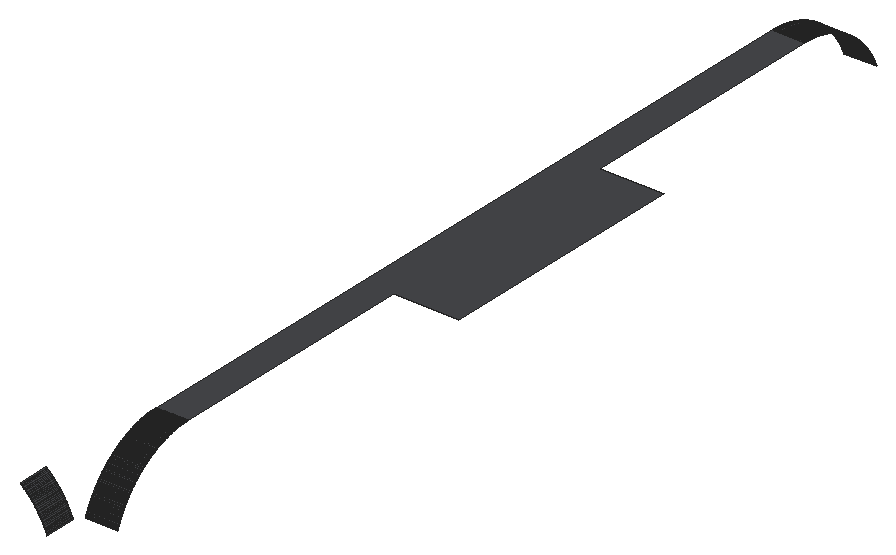
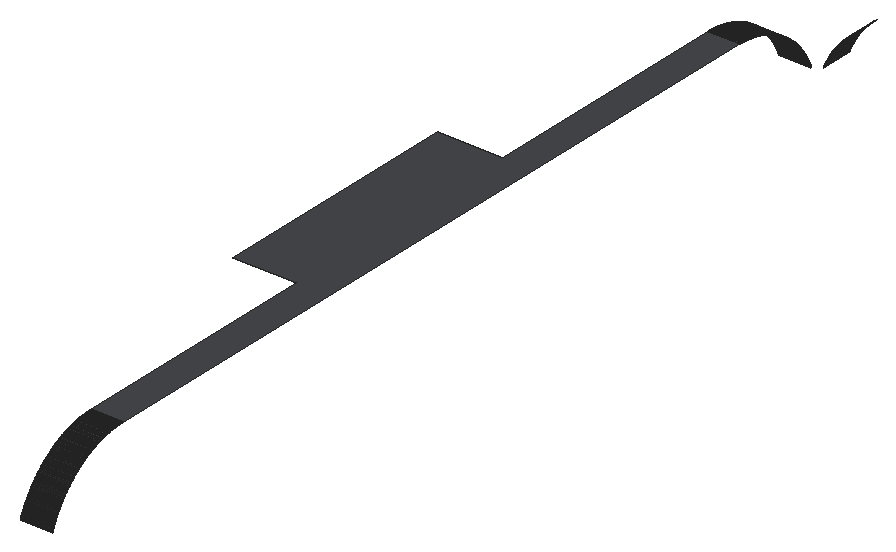
# SketchUp Ruby script. Lengths in inches.
U = 1.inch
M = Sketchup.active_model
def pt(a) = Geom::Point3d.new(a.map { |v| v * U })
def face(e, loops, mat)
  f = e.add_face(loops[0].map { |a| pt(a) })
  loops[1..].each { |l| e.add_face(l.map { |a| pt(a) }).erase! }
  f.material = f.back_material = mat if mat
  f
end
# faces: each face lists its corners as indices into pts; further lists are holes
def faces(e, pts, list, mat = nil) = list.each { |f| face(e, (f[0].is_a?(Array) ? f : [f]).map { |l| l.map { |i| pts[i] } }, mat) }
# xy, xz, yz: faces in a plane at the given z, y or x. An outline is a flat list of corners, or four numbers for a rectangle; further outlines are holes
def ring(l) = l.size == 4 ? [[l[0], l[1]], [l[2], l[1]], [l[2], l[3]], [l[0], l[3]]] : l.each_slice(2).to_a
def flat(e, list, mat, &to3) = list.each { |f| face(e, (f[0].is_a?(Array) ? f : [f]).map { |l| ring(l).map { |u, v| to3.(u, v) } }, mat) }
def xy(e, z, list, mat = nil) = flat(e, list, mat) { |x, y| [x, y, z] }
def xz(e, y, list, mat = nil) = flat(e, list, mat) { |x, z| [x, y, z] }
def yz(e, x, list, mat = nil) = flat(e, list, mat) { |y, z| [x, y, z] }
def lines(e, pts, list) = list.each { |a, b| e.add_line(pt(pts[a]), pt(pts[b])) }
# prism: a flat outline (further loops are holes) pulled along v
def prism(e, loops, v, mat = nil)
  f = face(e, loops, mat); d = Geom::Vector3d.new(v.map { |x| x * U })
  f.pushpull(f.normal.samedirection?(d) ? d.length : -d.length)
end
def box(e, o, s, mat = nil) = prism(e, [[o, [o[0] + s[0], o[1], o[2]], [o[0] + s[0], o[1] + s[1], o[2]], [o[0], o[1] + s[1], o[2]]]], [0, 0, s[2]], mat)
def at(x, y, z, deg = 0) = Geom::Transformation.translation(pt([x, y, z])) * Geom::Transformation.rotation(ORIGIN, Z_AXIS, deg.degrees)
def axes(o, x, y, z) = Geom::Transformation.new([*x, 0, *y, 0, *z, 0, *pt(o).to_a, 1])
def part(name) = M.definitions.add(name)
# library, detail: a bought-in or finely detailed component or shape, given as its bounding box
def library(name, o, s) = part(name).tap { |d| box(d.entities, o, s) }
def detail(e, o, s) = box(e.add_group.entities, o, s)
def put(e, d, t, mat = nil) = e.add_instance(d, t).tap { |i| i.material = mat if mat }
def group(e, t, mat = nil) = e.add_group.tap { |g| g.transformation = t; g.material = mat if mat }.entities
root = M.entities
M.materials.add("1432 AP 8245 TAR ROAD").color = [71, 72, 75]
xy(root,596.79,[[573,142.8,585,143.09],[573,143.09,585,143.37],[573,143.37,585,143.37,585,239.37,609,239.37,609,335.37,585,335.37,585,431.37,573,431.37],[573,431.37,585,431.65],[573,431.65,585,431.94]],"1432 AP 8245 TAR ROAD")
p = [[570.47,107.37,574.04],[570.37,107.37,574.31],[570.37,95.37,574.31],[570.47,95.37,574.04],[570.26,107.37,574.57],[570.26,95.37,574.57],
  [573,110.11,574.57],[573,110,574.31],[585,110,574.31],[585,110.11,574.57],[573,464.74,574.31],[573,464.63,574.57],
  [585,464.63,574.57],[585,464.74,574.31],[570.15,107.37,574.83],[570.15,95.37,574.83],[573,110.22,574.83],[585,110.22,574.83],
  [573,464.52,574.83],[585,464.52,574.83],[570.04,107.37,575.09],[570.04,95.37,575.09],[573,110.33,575.09],[585,110.33,575.09],
  [573,464.41,575.09],[585,464.41,575.09],[569.93,107.37,575.35],[569.93,95.37,575.35],[573,110.44,575.35],[585,110.44,575.35],
  [573,464.3,575.35],[585,464.3,575.35],[569.8125,107.37,575.61],[569.8125,95.37,575.61],[573,110.56,575.61],[585,110.56,575.61],
  [573,464.18,575.61],[585,464.18,575.61],[569.69,107.37,575.86],[569.69,95.37,575.86],[573,110.68,575.86],[585,110.68,575.86],
  [573,464.0625,575.86],[585,464.0625,575.86],[569.57,107.37,576.12],[569.57,95.37,576.12],[573,110.8,576.12],[585,110.8,576.12],
  [573,463.94,576.12],[585,463.94,576.12],[569.45,107.37,576.375],[569.45,95.37,576.375],[573,110.92,576.375],[585,110.92,576.375],
  [573,463.82,576.375],[585,463.82,576.375],[569.33,107.37,576.63],[569.33,95.37,576.63],[573,111.04,576.63],[585,111.04,576.63],
  [573,463.7,576.63],[585,463.7,576.63],[569.2,107.37,576.88],[569.2,95.37,576.88],[573,111.17,576.88],[585,111.17,576.88],
  [573,463.57,576.88],[585,463.57,576.88],[569.08,107.37,577.14],[569.08,95.37,577.14],[573,111.29,577.14],[585,111.29,577.14],
  [573,463.45,577.14],[585,463.45,577.14],[568.95,107.37,577.39],[568.95,95.37,577.39],[573,111.42,577.39],[585,111.42,577.39],
  [573,463.32,577.39],[585,463.32,577.39],[568.82,107.37,577.64],[568.82,95.37,577.64],[573,111.55,577.64],[585,111.55,577.64],
  [573,463.19,577.64],[585,463.19,577.64],[568.68,107.37,577.89],[568.68,95.37,577.89],[573,111.6875,577.89],[585,111.6875,577.89],
  [573,463.05,577.89],[585,463.05,577.89],[568.55,107.37,578.14],[568.55,95.37,578.14],[573,111.82,578.14],[585,111.82,578.14],
  [573,462.92,578.14],[585,462.92,578.14],[568.41,107.37,578.38],[568.41,95.37,578.38],[573,111.96,578.38],[585,111.96,578.38],
  [573,462.78,578.38],[585,462.78,578.38],[568.27,107.37,578.63],[568.27,95.37,578.63],[573,112.1,578.63],[585,112.1,578.63],
  [573,462.64,578.63],[585,462.64,578.63],[568.13,107.37,578.875],[568.13,95.37,578.875],[573,112.24,578.875],[585,112.24,578.875],
  [573,462.5,578.875],[585,462.5,578.875],[567.99,107.37,579.12],[567.99,95.37,579.12],[573,112.38,579.12],[585,112.38,579.12],
  [573,462.36,579.12],[585,462.36,579.12],[567.84,107.37,579.36],[567.84,95.37,579.36],[573,112.53,579.36],[585,112.53,579.36],
  [573,462.21,579.36],[585,462.21,579.36],[567.7,107.37,579.6],[567.7,95.37,579.6],[573,112.67,579.6],[585,112.67,579.6],
  [573,462.06,579.6],[585,462.06,579.6],[567.55,107.37,579.84],[567.55,95.37,579.84],[573,112.82,579.84],[585,112.82,579.84],
  [573,461.92,579.84],[585,461.92,579.84],[567.4,107.37,580.08],[567.4,95.37,580.08],[573,112.97,580.08],[585,112.97,580.08],
  [573,461.77,580.08],[585,461.77,580.08],[567.24,107.37,580.32],[567.24,95.37,580.32],[573,113.125,580.32],[585,113.125,580.32],
  [573,461.61,580.32],[585,461.61,580.32],[567.09,107.37,580.56],[567.09,95.37,580.56],[573,113.28,580.56],[585,113.28,580.56],
  [573,461.46,580.56],[585,461.46,580.56],[566.93,107.37,580.79],[566.93,95.37,580.79],[573,113.4375,580.79],[585,113.4375,580.79],
  [573,461.3,580.79],[585,461.3,580.79],[566.77,107.37,581.03],[566.77,95.37,581.03],[573,113.6,581.03],[585,113.6,581.03],
  [573,461.14,581.03],[585,461.14,581.03],[566.62,107.37,581.26],[566.62,95.37,581.26],[573,113.75,581.26],[585,113.75,581.26],
  [573,460.98,581.26],[585,460.98,581.26],[566.45,107.37,581.49],[566.45,95.37,581.49],[573,113.92,581.49],[585,113.92,581.49],
  [573,460.82,581.49],[585,460.82,581.49],[566.29,107.37,581.72],[566.29,95.37,581.72],[573,114.08,581.72],[585,114.08,581.72],
  [573,460.66,581.72],[585,460.66,581.72],[566.125,107.37,581.95],[566.125,95.37,581.95],[573,114.25,581.95],[585,114.25,581.95],
  [573,460.49,581.95],[585,460.49,581.95],[565.96,107.37,582.18],[565.96,95.37,582.18],[573,114.41,582.18],[585,114.41,582.18],
  [573,460.33,582.18],[585,460.33,582.18],[565.79,107.37,582.41],[565.79,95.37,582.41],[573,114.58,582.41],[585,114.58,582.41],
  [573,460.16,582.41],[585,460.16,582.41],[565.62,107.37,582.63],[565.62,95.37,582.63],[573,114.75,582.63],[585,114.75,582.63],
  [573,459.99,582.63],[585,459.99,582.63],[565.45,107.37,582.86],[565.45,95.37,582.86],[573,114.92,582.86],[585,114.92,582.86],
  [573,459.82,582.86],[585,459.82,582.86],[565.27,107.37,583.08],[565.27,95.37,583.08],[573,115.1,583.08],[585,115.1,583.08],
  [573,459.64,583.08],[585,459.64,583.08],[565.1,107.37,583.3],[565.1,95.37,583.3],[573,115.27,583.3],[585,115.27,583.3],
  [573,459.47,583.3],[585,459.47,583.3],[564.92,107.37,583.52],[564.92,95.37,583.52],[573,115.45,583.52],[585,115.45,583.52],
  [573,459.29,583.52],[585,459.29,583.52],[564.74,107.37,583.74],[564.74,95.37,583.74],[573,115.63,583.74],[585,115.63,583.74],
  [573,459.11,583.74],[585,459.11,583.74],[564.56,107.37,583.96],[564.56,95.37,583.96],[573,115.8125,583.96],[585,115.8125,583.96],
  [573,458.93,583.96],[585,458.93,583.96],[564.375,107.37,584.17],[564.375,95.37,584.17],[573,116,584.17],[585,116,584.17],
  [573,458.74,584.17],[585,458.74,584.17],[564.19,107.37,584.39],[564.19,95.37,584.39],[573,116.18,584.39],[585,116.18,584.39],
  [573,458.56,584.39],[585,458.56,584.39],[564,107.37,584.6],[564,95.37,584.6],[573,116.37,584.6],[585,116.37,584.6],
  [573,458.375,584.6],[585,458.375,584.6],[563.82,107.37,584.8125],[563.82,95.37,584.8125],[573,116.55,584.8125],[585,116.55,584.8125],
  [573,458.1875,584.8125],[585,458.1875,584.8125],[563.625,107.37,585.02],[563.625,95.37,585.02],[573,116.74,585.02],[585,116.74,585.02],
  [573,458,585.02],[585,458,585.02],[563.4375,107.37,585.23],[563.4375,95.37,585.23],[573,116.93,585.23],[585,116.93,585.23],
  [573,457.81,585.23],[585,457.81,585.23],[563.24,107.37,585.4375],[563.24,95.37,585.4375],[573,117.13,585.4375],[585,117.13,585.4375],
  [573,457.61,585.4375],[585,457.61,585.4375],[563.05,107.37,585.64],[563.05,95.37,585.64],[573,117.32,585.64],[585,117.32,585.64],
  [573,457.42,585.64],[585,457.42,585.64],[562.85,107.37,585.84],[562.85,95.37,585.84],[573,117.52,585.84],[585,117.52,585.84],
  [573,457.22,585.84],[585,457.22,585.84],[562.65,107.37,586.05],[562.65,95.37,586.05],[573,117.71,586.05],[585,117.71,586.05],
  [573,457.02,586.05],[585,457.02,586.05],[562.46,107.37,586.25],[562.46,95.37,586.25],[573,117.91,586.25],[585,117.91,586.25],
  [573,456.83,586.25],[585,456.83,586.25],[562.26,107.37,586.45],[562.26,95.37,586.45],[573,118.11,586.45],[585,118.11,586.45],
  [573,456.625,586.45],[585,456.625,586.45],[562.05,107.37,586.64],[562.05,95.37,586.64],[573,118.32,586.64],[585,118.32,586.64],
  [573,456.42,586.64],[585,456.42,586.64],[561.85,107.37,586.84],[561.85,95.37,586.84],[573,118.52,586.84],[585,118.52,586.84],
  [573,456.22,586.84],[585,456.22,586.84],[561.64,107.37,587.03],[561.64,95.37,587.03],[573,118.73,587.03],[585,118.73,587.03],
  [573,456.01,587.03],[585,456.01,587.03],[561.4375,107.37,587.23],[561.4375,95.37,587.23],[573,118.93,587.23],[585,118.93,587.23],
  [573,455.81,587.23],[585,455.81,587.23],[561.23,107.37,587.42],[561.23,95.37,587.42],[573,119.14,587.42],[585,119.14,587.42],
  [573,455.6,587.42],[585,455.6,587.42],[561.02,107.37,587.61],[561.02,95.37,587.61],[573,119.35,587.61],[585,119.35,587.61],
  [573,455.39,587.61],[585,455.39,587.61],[560.81,107.37,587.8],[560.81,95.37,587.8],[573,119.5625,587.8],[585,119.5625,587.8],
  [573,455.18,587.8],[585,455.18,587.8],[560.59,107.37,587.98],[560.59,95.37,587.98],[573,119.78,587.98],[585,119.78,587.98],
  [573,454.96,587.98],[585,454.96,587.98],[560.38,107.37,588.17],[560.38,95.37,588.17],[573,119.99,588.17],[585,119.99,588.17],
  [573,454.75,588.17],[585,454.75,588.17],[573,120.21,588.35],[585,120.21,588.35],[573,454.53,588.35],[585,454.53,588.35],
  [573,120.42,588.53],[585,120.42,588.53],[573,454.32,588.53],[585,454.32,588.53],[573,120.64,588.71],[585,120.64,588.71],
  [573,454.1,588.71],[585,454.1,588.71],[573,120.86,588.89],[585,120.86,588.89],[573,453.88,588.89],[585,453.88,588.89],
  [573,121.08,589.0625],[585,121.08,589.0625],[573,453.66,589.0625],[585,453.66,589.0625],[573,121.31,589.24],[585,121.31,589.24],
  [573,453.43,589.24],[585,453.43,589.24],[573,121.53,589.41],[585,121.53,589.41],[573,453.21,589.41],[585,453.21,589.41],
  [573,121.75,589.58],[585,121.75,589.58],[573,452.99,589.58],[585,452.99,589.58],[573,121.98,589.75],[585,121.98,589.75],
  [573,452.76,589.75],[585,452.76,589.75],[573,122.21,589.92],[585,122.21,589.92],[573,452.53,589.92],[585,452.53,589.92],
  [573,122.4375,590.08],[585,122.4375,590.08],[573,452.3,590.08],[585,452.3,590.08],[573,122.67,590.25],[585,122.67,590.25],
  [573,452.07,590.25],[585,452.07,590.25],[573,122.9,590.41],[585,122.9,590.41],[573,451.84,590.41],[585,451.84,590.41],
  [573,123.13,590.57],[585,123.13,590.57],[573,451.6,590.57],[585,451.6,590.57],[573,123.37,590.72],[585,123.37,590.72],
  [573,451.37,590.72],[585,451.37,590.72],[573,123.61,590.88],[585,123.61,590.88],[573,451.13,590.88],[585,451.13,590.88],
  [573,123.84,591.04],[585,123.84,591.04],[573,450.9,591.04],[585,450.9,591.04],[573,124.08,591.1875],[585,124.08,591.1875],
  [573,450.66,591.1875],[585,450.66,591.1875],[573,124.32,591.34],[585,124.32,591.34],[573,450.42,591.34],[585,450.42,591.34],
  [573,124.56,591.49],[585,124.56,591.49],[573,450.18,591.49],[585,450.18,591.49],[573,124.8,591.63],[585,124.8,591.63],
  [573,449.9375,591.63],[585,449.9375,591.63],[573,125.04,591.78],[585,125.04,591.78],[573,449.7,591.78],[585,449.7,591.78],
  [573,125.29,591.92],[585,125.29,591.92],[573,449.45,591.92],[585,449.45,591.92],[573,125.53,592.0625],[585,125.53,592.0625],
  [573,449.21,592.0625],[585,449.21,592.0625],[573,125.78,592.2],[585,125.78,592.2],[573,448.96,592.2],[585,448.96,592.2],
  [573,126.03,592.34],[585,126.03,592.34],[573,448.71,592.34],[585,448.71,592.34],[573,126.28,592.47],[585,126.28,592.47],
  [573,448.46,592.47],[585,448.46,592.47],[573,126.52,592.61],[585,126.52,592.61],[573,448.22,592.61],[585,448.22,592.61],
  [573,126.77,592.74],[585,126.77,592.74],[573,447.97,592.74],[585,447.97,592.74],[573,127.03,592.87],[585,127.03,592.87],
  [573,447.71,592.87],[585,447.71,592.87],[573,127.28,593],[585,127.28,593],[573,447.46,593],[585,447.46,593],
  [573,127.53,593.12],[585,127.53,593.12],[573,447.21,593.12],[585,447.21,593.12],[573,127.79,593.24],[585,127.79,593.24],
  [573,446.95,593.24],[585,446.95,593.24],[573,128.04,593.37],[585,128.04,593.37],[573,446.7,593.37],[585,446.7,593.37],
  [573,128.3,593.49],[585,128.3,593.49],[573,446.44,593.49],[585,446.44,593.49],[573,128.56,593.6],[585,128.56,593.6],
  [573,446.18,593.6],[585,446.18,593.6],[573,128.8125,593.72],[585,128.8125,593.72],[573,445.93,593.72],[585,445.93,593.72],
  [573,129.07,593.83],[585,129.07,593.83],[573,445.67,593.83],[585,445.67,593.83],[573,129.33,593.94],[585,129.33,593.94],
  [573,445.41,593.94],[585,445.41,593.94],[573,129.59,594.05],[585,129.59,594.05],[573,445.15,594.05],[585,445.15,594.05],
  [573,129.85,594.16],[585,129.85,594.16],[573,444.88,594.16],[585,444.88,594.16],[573,130.12,594.26],[585,130.12,594.26],
  [573,444.62,594.26],[585,444.62,594.26],[573,130.38,594.37],[585,130.38,594.37],[573,444.36,594.37],[585,444.36,594.37],
  [573,130.64,594.47],[585,130.64,594.47],[573,444.1,594.47],[585,444.1,594.47],[573,130.91,594.57],[585,130.91,594.57],
  [573,443.83,594.57],[585,443.83,594.57],[573,131.18,594.66],[585,131.18,594.66],[573,443.5625,594.66],[585,443.5625,594.66],
  [573,131.44,594.76],[585,131.44,594.76],[573,443.3,594.76],[585,443.3,594.76],[573,131.71,594.85],[585,131.71,594.85],
  [573,443.03,594.85],[585,443.03,594.85],[573,131.98,594.94],[585,131.98,594.94],[573,132.25,595.03],[585,132.25,595.03],
  [573,442.76,594.94],[573,442.49,595.03],[585,442.49,595.03],[585,442.76,594.94],[573,132.51,595.12],[585,132.51,595.12],
  [573,442.23,595.12],[585,442.23,595.12],[573,132.78,595.2],[585,132.78,595.2],[573,441.96,595.2],[585,441.96,595.2],
  [573,133.06,595.28],[585,133.06,595.28],[573,441.68,595.28],[585,441.68,595.28],[573,133.33,595.36],[585,133.33,595.36],
  [573,441.41,595.36],[585,441.41,595.36],[573,133.6,595.44],[585,133.6,595.44],[573,133.87,595.52],[585,133.87,595.52],
  [573,441.14,595.44],[573,440.87,595.52],[585,440.87,595.52],[585,441.14,595.44],[573,134.14,595.59],[585,134.14,595.59],
  [573,440.6,595.59],[585,440.6,595.59],[573,134.42,595.66],[585,134.42,595.66],[573,440.32,595.66],[585,440.32,595.66],
  [573,134.69,595.73],[585,134.69,595.73],[573,134.97,595.8],[585,134.97,595.8],[573,440.05,595.73],[573,439.77,595.8],
  [585,439.77,595.8],[585,440.05,595.73],[573,135.24,595.86],[585,135.24,595.86],[573,439.5,595.86],[585,439.5,595.86],
  [573,135.52,595.93],[585,135.52,595.93],[573,135.79,595.99],[585,135.79,595.99],[573,439.22,595.93],[573,438.95,595.99],
  [585,438.95,595.99],[585,439.22,595.93],[573,136.07,596.04],[585,136.07,596.04],[573,136.35,596.1],[585,136.35,596.1],
  [573,438.67,596.04],[573,438.39,596.1],[585,438.39,596.1],[585,438.67,596.04],[573,136.625,596.15],[585,136.625,596.15],
  [573,438.12,596.15],[585,438.12,596.15],[573,136.9,596.21],[585,136.9,596.21],[573,137.18,596.26],[585,137.18,596.26],
  [573,437.84,596.21],[573,437.56,596.26],[585,437.56,596.26],[585,437.84,596.21],[573,137.46,596.3],[585,137.46,596.3],
  [573,137.74,596.35],[585,137.74,596.35],[573,138.02,596.39],[585,138.02,596.39],[573,437,596.35],[573,436.72,596.39],
  [585,436.72,596.39],[585,437,596.35],[573,437.28,596.3],[585,437.28,596.3],[573,138.3,596.43],[585,138.3,596.43],
  [573,138.58,596.47],[585,138.58,596.47],[573,436.44,596.43],[573,436.16,596.47],[585,436.16,596.47],[585,436.44,596.43],
  [573,138.86,596.51],[585,138.86,596.51],[573,139.14,596.54],[585,139.14,596.54],[573,139.42,596.57],[585,139.42,596.57],
  [573,435.6,596.54],[573,435.32,596.57],[585,435.32,596.57],[585,435.6,596.54],[573,435.88,596.51],[585,435.88,596.51],
  [573,139.7,596.6],[585,139.7,596.6],[573,139.98,596.63],[585,139.98,596.63],[573,140.26,596.66],[585,140.26,596.66],
  [573,434.76,596.63],[573,434.48,596.66],[585,434.48,596.66],[585,434.76,596.63],[573,435.04,596.6],[585,435.04,596.6],
  [573,140.55,596.68],[585,140.55,596.68],[573,140.83,596.7],[585,140.83,596.7],[573,141.11,596.72],[585,141.11,596.72],
  [573,141.39,596.74],[585,141.39,596.74],[573,141.67,596.75],[585,141.67,596.75],[573,433.35,596.74],[573,433.07,596.75],
  [585,433.07,596.75],[585,433.35,596.74],[573,433.63,596.72],[585,433.63,596.72],[573,433.91,596.7],[585,433.91,596.7],
  [573,434.19,596.68],[585,434.19,596.68],[573,141.96,596.76],[585,141.96,596.76],[573,142.24,596.77],[585,142.24,596.77],
  [573,142.52,596.78],[585,142.52,596.78],[573,142.8,596.79],[585,142.8,596.79],[573,432.22,596.78],[573,431.94,596.79],
  [585,431.94,596.79],[585,432.22,596.78],[573,432.5,596.77],[585,432.5,596.77],[573,432.78,596.76],[585,432.78,596.76]]
faces(root,p,[[0,1,2,3],[1,4,5,2],[6,7,8,9],[10,11,12,13],[4,14,15,5],[16,6,9,17],[11,18,19,12],[14,20,21,15],
  [22,16,17,23],[18,24,25,19],[20,26,27,21],[28,22,23,29],[24,30,31,25],[26,32,33,27],[34,28,29,35],[30,36,37,31],
  [32,38,39,33],[40,34,35,41],[36,42,43,37],[38,44,45,39],[46,40,41,47],[42,48,49,43],[44,50,51,45],[52,46,47,53],
  [48,54,55,49],[50,56,57,51],[58,52,53,59],[54,60,61,55],[56,62,63,57],[64,58,59,65],[60,66,67,61],[62,68,69,63],
  [70,64,65,71],[66,72,73,67],[68,74,75,69],[76,70,71,77],[72,78,79,73],[74,80,81,75],[82,76,77,83],[78,84,85,79],
  [80,86,87,81],[88,82,83,89],[84,90,91,85],[86,92,93,87],[94,88,89,95],[90,96,97,91],[92,98,99,93],[100,94,95,101],
  [96,102,103,97],[98,104,105,99],[106,100,101,107],[102,108,109,103],[104,110,111,105],[112,106,107,113],[108,114,115,109],[110,116,117,111],
  [118,112,113,119],[114,120,121,115],[116,122,123,117],[124,118,119,125],[120,126,127,121],[122,128,129,123],[130,124,125,131],[126,132,133,127],
  [128,134,135,129],[136,130,131,137],[132,138,139,133],[134,140,141,135],[142,136,137,143],[138,144,145,139],[140,146,147,141],[148,142,143,149],
  [144,150,151,145],[146,152,153,147],[154,148,149,155],[150,156,157,151],[152,158,159,153],[160,154,155,161],[156,162,163,157],[158,164,165,159],
  [166,160,161,167],[162,168,169,163],[164,170,171,165],[172,166,167,173],[168,174,175,169],[170,176,177,171],[178,172,173,179],[174,180,181,175],
  [176,182,183,177],[184,178,179,185],[180,186,187,181],[182,188,189,183],[190,184,185,191],[186,192,193,187],[188,194,195,189],[196,190,191,197],
  [192,198,199,193],[194,200,201,195],[202,196,197,203],[198,204,205,199],[200,206,207,201],[208,202,203,209],[204,210,211,205],[206,212,213,207],
  [214,208,209,215],[210,216,217,211],[212,218,219,213],[220,214,215,221],[216,222,223,217],[218,224,225,219],[226,220,221,227],[222,228,229,223],
  [224,230,231,225],[232,226,227,233],[228,234,235,229],[230,236,237,231],[238,232,233,239],[234,240,241,235],[236,242,243,237],[244,238,239,245],
  [240,246,247,241],[242,248,249,243],[250,244,245,251],[246,252,253,247],[248,254,255,249],[256,250,251,257],[252,258,259,253],[254,260,261,255],
  [262,256,257,263],[258,264,265,259],[260,266,267,261],[268,262,263,269],[264,270,271,265],[266,272,273,267],[274,268,269,275],[270,276,277,271],
  [272,278,279,273],[280,274,275,281],[276,282,283,277],[278,284,285,279],[286,280,281,287],[282,288,289,283],[284,290,291,285],[292,286,287,293],
  [288,294,295,289],[290,296,297,291],[298,292,293,299],[294,300,301,295],[296,302,303,297],[304,298,299,305],[300,306,307,301],[302,308,309,303],
  [310,304,305,311],[306,312,313,307],[308,314,315,309],[316,310,311,317],[312,318,319,313],[314,320,321,315],[322,316,317,323],[318,324,325,319],
  [320,326,327,321],[328,322,323,329],[324,330,331,325],[326,332,333,327],[334,328,329,335],[330,336,337,331],[332,338,339,333],[340,334,335,341],
  [336,342,343,337],[338,344,345,339],[346,340,341,347],[342,348,349,343],[344,350,351,345],[352,346,347,353],[348,354,355,349],[350,356,357,351],
  [358,352,353,359],[354,360,361,355],[356,362,363,357],[364,358,359,365],[360,366,367,361],[362,368,369,363],[370,364,365,371],[366,372,373,367],
  [374,370,371,375],[372,376,377,373],[378,374,375,379],[376,380,381,377],[382,378,379,383],[380,384,385,381],[386,382,383,387],[384,388,389,385],
  [390,386,387,391],[388,392,393,389],[394,390,391,395],[392,396,397,393],[398,394,395,399],[396,400,401,397],[402,398,399,403],[400,404,405,401],
  [406,402,403,407],[404,408,409,405],[410,406,407,411],[408,412,413,409],[414,410,411,415],[412,416,417,413],[418,414,415,419],[416,420,421,417],
  [422,418,419,423],[420,424,425,421],[426,422,423,427],[424,428,429,425],[430,426,427,431],[428,432,433,429],[434,430,431,435],[432,436,437,433],
  [438,434,435,439],[436,440,441,437],[442,438,439,443],[440,444,445,441],[446,442,443,447],[444,448,449,445],[450,446,447,451],[448,452,453,449],
  [454,450,451,455],[452,456,457,453],[458,454,455,459],[456,460,461,457],[462,458,459,463],[460,464,465,461],[466,462,463,467],[464,468,469,465],
  [470,466,467,471],[468,472,473,469],[474,470,471,475],[472,476,477,473],[478,474,475,479],[476,480,481,477],[482,478,479,483],[480,484,485,481],
  [486,482,483,487],[484,488,489,485],[490,486,487,491],[488,492,493,489],[494,490,491,495],[492,496,497,493],[498,494,495,499],[496,500,501,497],
  [502,498,499,503],[500,504,505,501],[506,502,503,507],[504,508,509,505],[510,506,507,511],[508,512,513,509],[514,510,511,515],[512,516,517,513],
  [518,514,515,519],[516,520,521,517],[522,518,519,523],[520,524,525,521],[526,522,523,527],[524,528,529,525],[530,526,527,531],[528,532,533,529],
  [534,530,531,535],[532,536,537,533],[538,534,535,539],[536,540,541,537],[542,538,539,543],[540,544,545,541],[546,542,543,547],[544,548,549,545],
  [550,546,547,551],[548,552,553,549],[554,550,551,555],[552,556,557,553],[558,554,555,559],[556,560,561,557],[562,558,559,563],[560,564,565,561],
  [566,562,563,567],[568,566,567,569],[570,571,572,573],[564,570,573,565],[574,568,569,575],[571,576,577,572],[578,574,575,579],[576,580,581,577],
  [582,578,579,583],[580,584,585,581],[586,582,583,587],[584,588,589,585],[590,586,587,591],[592,590,591,593],[594,595,596,597],[588,594,597,589],
  [598,592,593,599],[595,600,601,596],[602,598,599,603],[600,604,605,601],[606,602,603,607],[608,606,607,609],[610,611,612,613],[604,610,613,605],
  [614,608,609,615],[611,616,617,612],[618,614,615,619],[620,618,619,621],[622,623,624,625],[616,622,625,617],[626,620,621,627],[628,626,627,629],
  [630,631,632,633],[623,630,633,624],[634,628,629,635],[631,636,637,632],[638,634,635,639],[640,638,639,641],[642,643,644,645],[636,642,645,637],
  [646,640,641,647],[648,646,647,649],[650,648,649,651],[652,653,654,655],[656,652,655,657],[643,656,657,644],[658,650,651,659],[660,658,659,661],
  [662,663,664,665],[653,662,665,654],[666,660,661,667],[668,666,667,669],[670,668,669,671],[672,673,674,675],[676,672,675,677],[663,676,677,664],
  [678,670,671,679],[680,678,679,681],[682,680,681,683],[684,685,686,687],[688,684,687,689],[673,688,689,674],[690,682,683,691],[692,690,691,693],
  [694,692,693,695],[696,694,695,697],[698,696,697,699],[700,701,702,703],[704,700,703,705],[706,704,705,707],[708,706,707,709],[685,708,709,686],
  [710,698,699,711],[712,710,711,713],[714,712,713,715],[716,714,715,717],[718,719,720,721],[722,718,721,723],[724,722,723,725],[701,724,725,702]],"1432 AP 8245 TAR ROAD")
